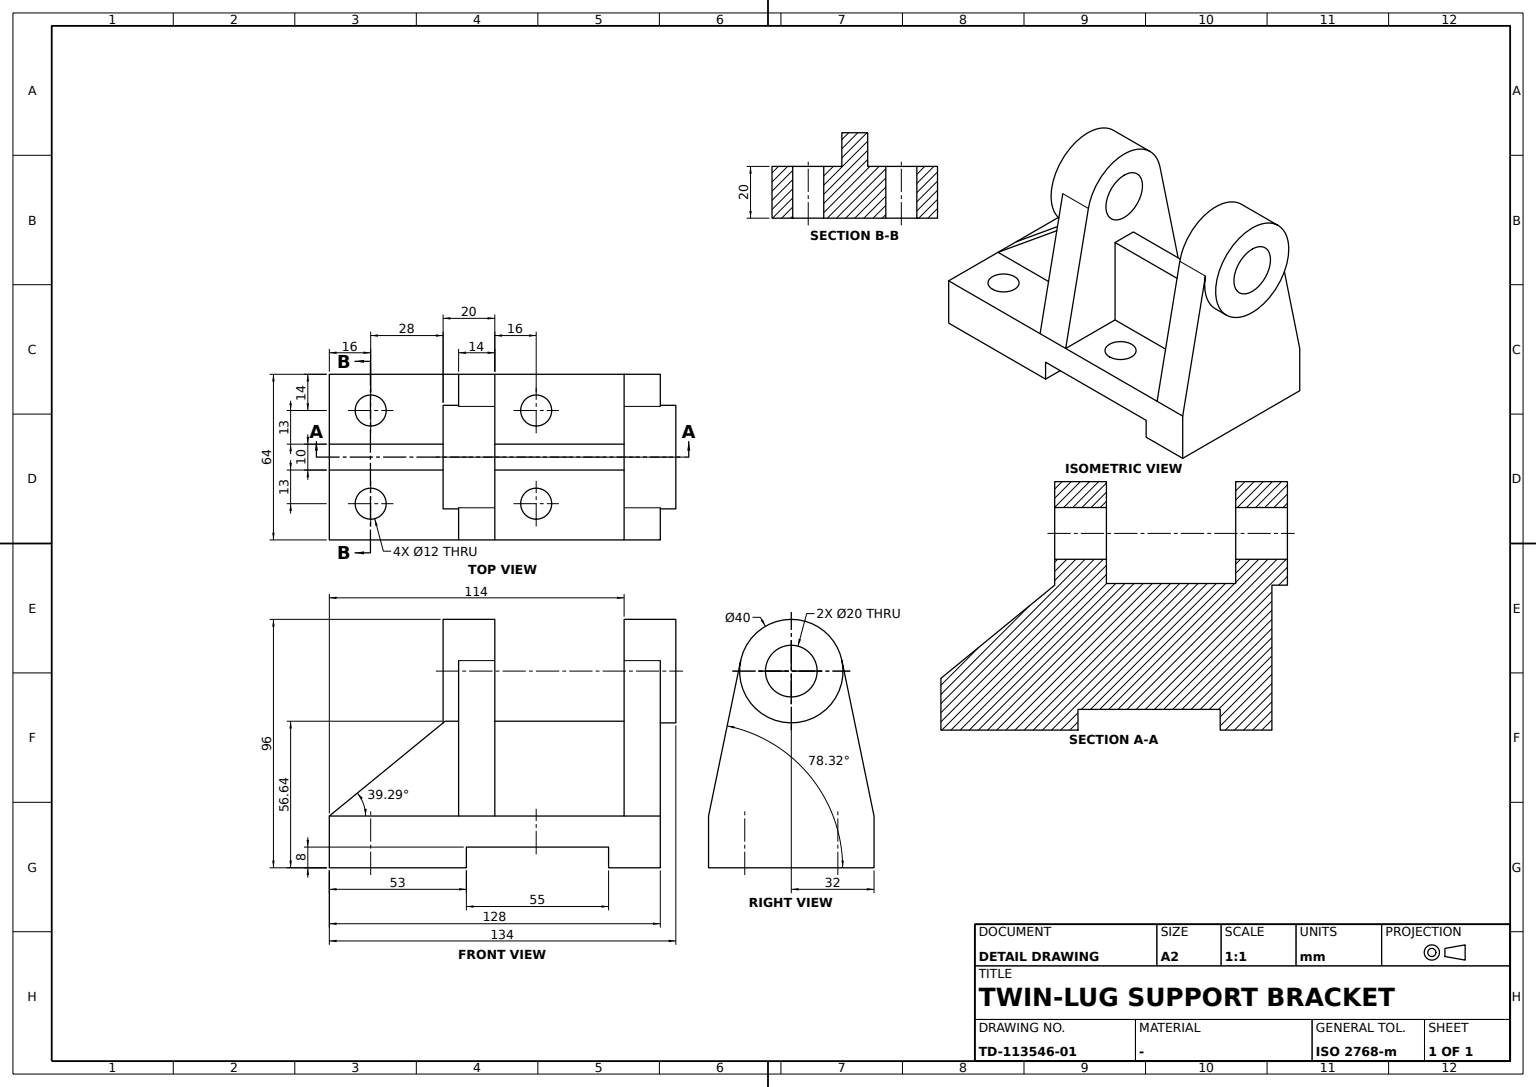
ISO-10303-21;
HEADER;
FILE_DESCRIPTION((''),'2;1');
FILE_NAME('','',(''),(''),'','','');
FILE_SCHEMA(('AUTOMOTIVE_DESIGN'));
ENDSEC;
DATA;
#1=APPLICATION_CONTEXT('');
#2=PRODUCT_CONTEXT('',#1,'mechanical');
#3=PRODUCT('','','',(#2));
#4=PRODUCT_DEFINITION_FORMATION('','',#3);
#5=PRODUCT_DEFINITION_CONTEXT('',#1,'design');
#6=PRODUCT_DEFINITION('','',#4,#5);
#7=PRODUCT_DEFINITION_SHAPE('','',#6);
#8=(LENGTH_UNIT()NAMED_UNIT(*)SI_UNIT(.MILLI.,.METRE.));
#9=(NAMED_UNIT(*)PLANE_ANGLE_UNIT()SI_UNIT($,.RADIAN.));
#10=(NAMED_UNIT(*)SI_UNIT($,.STERADIAN.)SOLID_ANGLE_UNIT());
#11=UNCERTAINTY_MEASURE_WITH_UNIT(LENGTH_MEASURE(0.005),#8,'distance_accuracy_value','');
#12=(GEOMETRIC_REPRESENTATION_CONTEXT(3)GLOBAL_UNCERTAINTY_ASSIGNED_CONTEXT((#11))GLOBAL_UNIT_ASSIGNED_CONTEXT((#8,#9,#10))REPRESENTATION_CONTEXT('',''));
#13=CARTESIAN_POINT('',(19.5858412334,50.,80.0490521334));
#14=VERTEX_POINT('',#13);
#15=CARTESIAN_POINT('',(19.5858412334,64.,80.0490521334));
#16=VERTEX_POINT('',#15);
#17=CARTESIAN_POINT('',(19.5858412334,60.,80.0490521334));
#18=DIRECTION('',(0.,1.,0.));
#19=VECTOR('',#18,1000.);
#20=LINE('',#17,#19);
#21=EDGE_CURVE('',#14,#16,#20,.T.);
#22=ORIENTED_EDGE('',*,*,#21,.T.);
#23=CARTESIAN_POINT('',(-19.5858412334,64.,80.0490521334));
#24=VERTEX_POINT('',#23);
#25=CARTESIAN_POINT('',(0.,64.,76.));
#26=DIRECTION('',(0.,0.,1.));
#27=AXIS2_PLACEMENT_3D('',#25,#18,#26);
#28=CIRCLE('',#27,20.);
#29=EDGE_CURVE('',#16,#24,#28,.T.);
#30=ORIENTED_EDGE('',*,*,#29,.T.);
#31=CARTESIAN_POINT('',(-19.5858412334,50.,80.0490521334));
#32=VERTEX_POINT('',#31);
#33=CARTESIAN_POINT('',(-19.5858412334,60.,80.0490521334));
#34=LINE('',#33,#19);
#35=EDGE_CURVE('',#32,#24,#34,.T.);
#36=ORIENTED_EDGE('',*,*,#35,.F.);
#37=CARTESIAN_POINT('',(0.,50.,76.));
#38=AXIS2_PLACEMENT_3D('',#37,#18,#26);
#39=CIRCLE('',#38,20.);
#40=EDGE_CURVE('',#32,#14,#39,.T.);
#41=ORIENTED_EDGE('',*,*,#40,.T.);
#42=EDGE_LOOP('',(#22,#30,#36,#41));
#43=FACE_BOUND('',#42,.T.);
#44=CARTESIAN_POINT('',(0.,70.,96.));
#45=VERTEX_POINT('',#44);
#46=CARTESIAN_POINT('',(0.,70.,76.));
#47=AXIS2_PLACEMENT_3D('',#46,#18,#26);
#48=CIRCLE('',#47,20.);
#49=EDGE_CURVE('',#45,#45,#48,.T.);
#50=ORIENTED_EDGE('',*,*,#49,.F.);
#51=EDGE_LOOP('',(#50));
#52=FACE_BOUND('',#51,.T.);
#53=CARTESIAN_POINT('',(0.,60.,76.));
#54=DIRECTION('',(-1.,0.,0.));
#55=AXIS2_PLACEMENT_3D('',#53,#18,#54);
#56=CYLINDRICAL_SURFACE('',#55,20.);
#57=ADVANCED_FACE('',(#43,#52),#56,.T.);
#58=CARTESIAN_POINT('',(-32.,44.,0.));
#59=VERTEX_POINT('',#58);
#60=CARTESIAN_POINT('',(32.,44.,0.));
#61=VERTEX_POINT('',#60);
#62=CARTESIAN_POINT('',(0.,44.,0.));
#63=DIRECTION('',(1.,0.,0.));
#64=VECTOR('',#63,1000.);
#65=LINE('',#62,#64);
#66=EDGE_CURVE('',#59,#61,#65,.T.);
#67=ORIENTED_EDGE('',*,*,#66,.T.);
#68=CARTESIAN_POINT('',(32.,44.,8.));
#69=VERTEX_POINT('',#68);
#70=VECTOR('',#26,1000.);
#71=LINE('',#60,#70);
#72=EDGE_CURVE('',#61,#69,#71,.T.);
#73=ORIENTED_EDGE('',*,*,#72,.T.);
#74=CARTESIAN_POINT('',(-32.,44.,8.));
#75=VERTEX_POINT('',#74);
#76=CARTESIAN_POINT('',(0.,44.,8.));
#77=LINE('',#76,#64);
#78=EDGE_CURVE('',#75,#69,#77,.T.);
#79=ORIENTED_EDGE('',*,*,#78,.F.);
#80=LINE('',#58,#70);
#81=EDGE_CURVE('',#59,#75,#80,.T.);
#82=ORIENTED_EDGE('',*,*,#81,.F.);
#83=EDGE_LOOP('',(#67,#73,#79,#82));
#84=FACE_BOUND('',#83,.T.);
#85=AXIS2_PLACEMENT_3D('',#62,#18,#26);
#86=PLANE('',#85);
#87=ADVANCED_FACE('',(#84),#86,.F.);
#88=CARTESIAN_POINT('',(-32.,-64.,20.));
#89=VERTEX_POINT('',#88);
#90=CARTESIAN_POINT('',(-32.,-64.,0.));
#91=VERTEX_POINT('',#90);
#92=DIRECTION('',(0.,0.,-1.));
#93=VECTOR('',#92,1000.);
#94=LINE('',#90,#93);
#95=EDGE_CURVE('',#89,#91,#94,.T.);
#96=ORIENTED_EDGE('',*,*,#95,.T.);
#97=CARTESIAN_POINT('',(32.,-64.,0.));
#98=VERTEX_POINT('',#97);
#99=CARTESIAN_POINT('',(0.,-64.,0.));
#100=LINE('',#99,#64);
#101=EDGE_CURVE('',#91,#98,#100,.T.);
#102=ORIENTED_EDGE('',*,*,#101,.T.);
#103=CARTESIAN_POINT('',(32.,-64.,20.));
#104=VERTEX_POINT('',#103);
#105=LINE('',#97,#93);
#106=EDGE_CURVE('',#104,#98,#105,.T.);
#107=ORIENTED_EDGE('',*,*,#106,.F.);
#108=CARTESIAN_POINT('',(5.,-64.,20.));
#109=VERTEX_POINT('',#108);
#110=CARTESIAN_POINT('',(0.,-64.,20.));
#111=LINE('',#110,#64);
#112=EDGE_CURVE('',#109,#104,#111,.T.);
#113=ORIENTED_EDGE('',*,*,#112,.F.);
#114=CARTESIAN_POINT('',(-5.,-64.,20.));
#115=VERTEX_POINT('',#114);
#116=EDGE_CURVE('',#115,#109,#111,.T.);
#117=ORIENTED_EDGE('',*,*,#116,.F.);
#118=EDGE_CURVE('',#89,#115,#111,.T.);
#119=ORIENTED_EDGE('',*,*,#118,.F.);
#120=EDGE_LOOP('',(#96,#102,#107,#113,#117,#119));
#121=FACE_BOUND('',#120,.T.);
#122=DIRECTION('',(0.,-1.,0.));
#123=AXIS2_PLACEMENT_3D('',#110,#122,#92);
#124=PLANE('',#123);
#125=ADVANCED_FACE('',(#121),#124,.T.);
#126=CARTESIAN_POINT('',(-5.,0.,20.));
#127=VERTEX_POINT('',#126);
#128=CARTESIAN_POINT('',(-32.,0.,20.));
#129=VERTEX_POINT('',#128);
#130=CARTESIAN_POINT('',(0.,0.,20.));
#131=VECTOR('',#54,1000.);
#132=LINE('',#130,#131);
#133=EDGE_CURVE('',#127,#129,#132,.T.);
#134=ORIENTED_EDGE('',*,*,#133,.F.);
#135=CARTESIAN_POINT('',(-5.,50.,20.));
#136=VERTEX_POINT('',#135);
#137=VECTOR('',#122,1000.);
#138=LINE('',#126,#137);
#139=EDGE_CURVE('',#136,#127,#138,.T.);
#140=ORIENTED_EDGE('',*,*,#139,.F.);
#141=CARTESIAN_POINT('',(-32.,50.,20.));
#142=VERTEX_POINT('',#141);
#143=CARTESIAN_POINT('',(0.,50.,20.));
#144=LINE('',#143,#131);
#145=EDGE_CURVE('',#136,#142,#144,.T.);
#146=ORIENTED_EDGE('',*,*,#145,.T.);
#147=LINE('',#128,#137);
#148=EDGE_CURVE('',#142,#129,#147,.T.);
#149=ORIENTED_EDGE('',*,*,#148,.T.);
#150=EDGE_LOOP('',(#134,#140,#146,#149));
#151=FACE_BOUND('',#150,.T.);
#152=CARTESIAN_POINT('',(-12.,16.,20.));
#153=VERTEX_POINT('',#152);
#154=CARTESIAN_POINT('',(-18.,16.,20.));
#155=AXIS2_PLACEMENT_3D('',#154,#26,#63);
#156=CIRCLE('',#155,6.);
#157=EDGE_CURVE('',#153,#153,#156,.T.);
#158=ORIENTED_EDGE('',*,*,#157,.F.);
#159=EDGE_LOOP('',(#158));
#160=FACE_BOUND('',#159,.T.);
#161=CARTESIAN_POINT('',(0.,64.,20.));
#162=AXIS2_PLACEMENT_3D('',#161,#26,#122);
#163=PLANE('',#162);
#164=ADVANCED_FACE('',(#151,#160),#163,.T.);
#165=CARTESIAN_POINT('',(-5.,-14.,56.635083269));
#166=VERTEX_POINT('',#165);
#167=CARTESIAN_POINT('',(-19.5858412334,-14.,80.0490521334));
#168=VERTEX_POINT('',#167);
#169=CARTESIAN_POINT('',(0.,-14.,76.));
#170=AXIS2_PLACEMENT_3D('',#169,#18,#26);
#171=CIRCLE('',#170,20.);
#172=EDGE_CURVE('',#166,#168,#171,.T.);
#173=ORIENTED_EDGE('',*,*,#172,.T.);
#174=CARTESIAN_POINT('',(-32.,-14.,20.));
#175=VERTEX_POINT('',#174);
#176=DIRECTION('',(-0.2024526067,0.,-0.9792920617));
#177=VECTOR('',#176,1000.);
#178=LINE('',#167,#177);
#179=EDGE_CURVE('',#168,#175,#178,.T.);
#180=ORIENTED_EDGE('',*,*,#179,.T.);
#181=CARTESIAN_POINT('',(-5.,-14.,20.));
#182=VERTEX_POINT('',#181);
#183=CARTESIAN_POINT('',(0.,-14.,20.));
#184=LINE('',#183,#131);
#185=EDGE_CURVE('',#182,#175,#184,.T.);
#186=ORIENTED_EDGE('',*,*,#185,.F.);
#187=CARTESIAN_POINT('',(-5.,-14.,0.));
#188=LINE('',#187,#93);
#189=EDGE_CURVE('',#166,#182,#188,.T.);
#190=ORIENTED_EDGE('',*,*,#189,.F.);
#191=EDGE_LOOP('',(#173,#180,#186,#190));
#192=FACE_BOUND('',#191,.T.);
#193=CARTESIAN_POINT('',(0.,-14.,0.));
#194=AXIS2_PLACEMENT_3D('',#193,#18,#54);
#195=PLANE('',#194);
#196=ADVANCED_FACE('',(#192),#195,.F.);
#197=CARTESIAN_POINT('',(-32.,-11.,0.));
#198=VERTEX_POINT('',#197);
#199=CARTESIAN_POINT('',(32.,-11.,0.));
#200=VERTEX_POINT('',#199);
#201=CARTESIAN_POINT('',(0.,-11.,0.));
#202=LINE('',#201,#64);
#203=EDGE_CURVE('',#198,#200,#202,.T.);
#204=ORIENTED_EDGE('',*,*,#203,.F.);
#205=CARTESIAN_POINT('',(-32.,-11.,8.));
#206=VERTEX_POINT('',#205);
#207=LINE('',#197,#93);
#208=EDGE_CURVE('',#206,#198,#207,.T.);
#209=ORIENTED_EDGE('',*,*,#208,.F.);
#210=CARTESIAN_POINT('',(32.,-11.,8.));
#211=VERTEX_POINT('',#210);
#212=CARTESIAN_POINT('',(0.,-11.,8.));
#213=LINE('',#212,#64);
#214=EDGE_CURVE('',#206,#211,#213,.T.);
#215=ORIENTED_EDGE('',*,*,#214,.T.);
#216=LINE('',#199,#93);
#217=EDGE_CURVE('',#211,#200,#216,.T.);
#218=ORIENTED_EDGE('',*,*,#217,.T.);
#219=EDGE_LOOP('',(#204,#209,#215,#218));
#220=FACE_BOUND('',#219,.T.);
#221=AXIS2_PLACEMENT_3D('',#212,#122,#92);
#222=PLANE('',#221);
#223=ADVANCED_FACE('',(#220),#222,.F.);
#224=CARTESIAN_POINT('',(32.,-14.,20.));
#225=VERTEX_POINT('',#224);
#226=CARTESIAN_POINT('',(32.,0.,20.));
#227=LINE('',#226,#137);
#228=EDGE_CURVE('',#225,#104,#227,.T.);
#229=ORIENTED_EDGE('',*,*,#228,.F.);
#230=CARTESIAN_POINT('',(5.,-14.,20.));
#231=VERTEX_POINT('',#230);
#232=EDGE_CURVE('',#225,#231,#184,.T.);
#233=ORIENTED_EDGE('',*,*,#232,.T.);
#234=CARTESIAN_POINT('',(5.,0.,20.));
#235=LINE('',#234,#137);
#236=EDGE_CURVE('',#231,#109,#235,.T.);
#237=ORIENTED_EDGE('',*,*,#236,.T.);
#238=ORIENTED_EDGE('',*,*,#112,.T.);
#239=EDGE_LOOP('',(#229,#233,#237,#238));
#240=FACE_BOUND('',#239,.T.);
#241=CARTESIAN_POINT('',(24.,-48.,20.));
#242=VERTEX_POINT('',#241);
#243=CARTESIAN_POINT('',(18.,-48.,20.));
#244=AXIS2_PLACEMENT_3D('',#243,#26,#63);
#245=CIRCLE('',#244,6.);
#246=EDGE_CURVE('',#242,#242,#245,.T.);
#247=ORIENTED_EDGE('',*,*,#246,.F.);
#248=EDGE_LOOP('',(#247));
#249=FACE_BOUND('',#248,.T.);
#250=ADVANCED_FACE('',(#240,#249),#163,.T.);
#251=CARTESIAN_POINT('',(32.,64.,20.));
#252=VERTEX_POINT('',#251);
#253=CARTESIAN_POINT('',(32.,50.,20.));
#254=VERTEX_POINT('',#253);
#255=LINE('',#251,#137);
#256=EDGE_CURVE('',#252,#254,#255,.T.);
#257=ORIENTED_EDGE('',*,*,#256,.F.);
#258=DIRECTION('',(0.2024526067,0.,-0.9792920617));
#259=VECTOR('',#258,1000.);
#260=LINE('',#15,#259);
#261=EDGE_CURVE('',#16,#252,#260,.T.);
#262=ORIENTED_EDGE('',*,*,#261,.F.);
#263=ORIENTED_EDGE('',*,*,#21,.F.);
#264=LINE('',#13,#259);
#265=EDGE_CURVE('',#14,#254,#264,.T.);
#266=ORIENTED_EDGE('',*,*,#265,.T.);
#267=EDGE_LOOP('',(#257,#262,#263,#266));
#268=FACE_BOUND('',#267,.T.);
#269=DIRECTION('',(-0.9792920617,0.,-0.2024526067));
#270=AXIS2_PLACEMENT_3D('',#15,#269,#258);
#271=PLANE('',#270);
#272=ADVANCED_FACE('',(#268),#271,.F.);
#273=CARTESIAN_POINT('',(-12.,16.,8.));
#274=VERTEX_POINT('',#273);
#275=CARTESIAN_POINT('',(-18.,16.,8.));
#276=AXIS2_PLACEMENT_3D('',#275,#26,#63);
#277=CIRCLE('',#276,6.);
#278=EDGE_CURVE('',#274,#274,#277,.T.);
#279=ORIENTED_EDGE('',*,*,#278,.F.);
#280=EDGE_LOOP('',(#279));
#281=FACE_BOUND('',#280,.T.);
#282=ORIENTED_EDGE('',*,*,#157,.T.);
#283=EDGE_LOOP('',(#282));
#284=FACE_BOUND('',#283,.T.);
#285=CARTESIAN_POINT('',(-18.,16.,9.));
#286=AXIS2_PLACEMENT_3D('',#285,#26,#63);
#287=CYLINDRICAL_SURFACE('',#286,6.);
#288=ADVANCED_FACE('',(#281,#284),#287,.F.);
#289=ORIENTED_EDGE('',*,*,#172,.F.);
#290=CARTESIAN_POINT('',(-5.,-19.2237871157,56.635083269));
#291=VERTEX_POINT('',#290);
#292=CARTESIAN_POINT('',(-5.,-14.0000000001,56.635083269));
#293=LINE('',#292,#19);
#294=EDGE_CURVE('',#166,#291,#293,.F.);
#295=ORIENTED_EDGE('',*,*,#294,.T.);
#296=CARTESIAN_POINT('',(0.,-20.,56.));
#297=VERTEX_POINT('',#296);
#298=CARTESIAN_POINT('',(0.,4.4444444444,76.));
#299=DIRECTION('',(0.,0.6332377903,-0.7739572992));
#300=DIRECTION('',(0.,0.7739572992,0.6332377903));
#301=AXIS2_PLACEMENT_3D('',#298,#299,#300);
#302=ELLIPSE('',#301,31.5837120079,20.);
#303=EDGE_CURVE('',#291,#297,#302,.F.);
#304=ORIENTED_EDGE('',*,*,#303,.T.);
#305=CARTESIAN_POINT('',(0.,-20.,76.));
#306=AXIS2_PLACEMENT_3D('',#305,#18,#26);
#307=CIRCLE('',#306,20.);
#308=EDGE_CURVE('',#297,#297,#307,.T.);
#309=ORIENTED_EDGE('',*,*,#308,.T.);
#310=CARTESIAN_POINT('',(5.,-19.2237871157,56.635083269));
#311=VERTEX_POINT('',#310);
#312=EDGE_CURVE('',#297,#311,#302,.F.);
#313=ORIENTED_EDGE('',*,*,#312,.T.);
#314=CARTESIAN_POINT('',(5.,-14.,56.635083269));
#315=VERTEX_POINT('',#314);
#316=CARTESIAN_POINT('',(5.,-14.0000000001,56.635083269));
#317=LINE('',#316,#19);
#318=EDGE_CURVE('',#315,#311,#317,.F.);
#319=ORIENTED_EDGE('',*,*,#318,.F.);
#320=CARTESIAN_POINT('',(19.5858412334,-14.,80.0490521334));
#321=VERTEX_POINT('',#320);
#322=EDGE_CURVE('',#321,#315,#171,.T.);
#323=ORIENTED_EDGE('',*,*,#322,.F.);
#324=CARTESIAN_POINT('',(19.5858412334,0.,80.0490521334));
#325=VERTEX_POINT('',#324);
#326=EDGE_CURVE('',#321,#325,#20,.T.);
#327=ORIENTED_EDGE('',*,*,#326,.T.);
#328=CARTESIAN_POINT('',(-19.5858412334,0.,80.0490521334));
#329=VERTEX_POINT('',#328);
#330=CARTESIAN_POINT('',(0.,0.,76.));
#331=AXIS2_PLACEMENT_3D('',#330,#18,#26);
#332=CIRCLE('',#331,20.);
#333=EDGE_CURVE('',#329,#325,#332,.T.);
#334=ORIENTED_EDGE('',*,*,#333,.F.);
#335=EDGE_CURVE('',#168,#329,#34,.T.);
#336=ORIENTED_EDGE('',*,*,#335,.F.);
#337=EDGE_LOOP('',(#289,#295,#304,#309,#313,#319,#323,#327,#334,#336));
#338=FACE_BOUND('',#337,.T.);
#339=ADVANCED_FACE('',(#338),#56,.T.);
#340=VERTEX_POINT('',#234);
#341=CARTESIAN_POINT('',(5.,0.,56.635083269));
#342=VERTEX_POINT('',#341);
#343=CARTESIAN_POINT('',(5.,0.,0.));
#344=LINE('',#343,#70);
#345=EDGE_CURVE('',#340,#342,#344,.T.);
#346=ORIENTED_EDGE('',*,*,#345,.F.);
#347=CARTESIAN_POINT('',(5.,50.,20.));
#348=VERTEX_POINT('',#347);
#349=EDGE_CURVE('',#348,#340,#235,.T.);
#350=ORIENTED_EDGE('',*,*,#349,.F.);
#351=CARTESIAN_POINT('',(5.,50.,56.635083269));
#352=VERTEX_POINT('',#351);
#353=CARTESIAN_POINT('',(5.,50.,0.));
#354=LINE('',#353,#70);
#355=EDGE_CURVE('',#348,#352,#354,.T.);
#356=ORIENTED_EDGE('',*,*,#355,.T.);
#357=LINE('',#341,#19);
#358=EDGE_CURVE('',#342,#352,#357,.T.);
#359=ORIENTED_EDGE('',*,*,#358,.F.);
#360=EDGE_LOOP('',(#346,#350,#356,#359));
#361=FACE_BOUND('',#360,.T.);
#362=AXIS2_PLACEMENT_3D('',#343,#63,#18);
#363=PLANE('',#362);
#364=ADVANCED_FACE('',(#361),#363,.T.);
#365=ORIENTED_EDGE('',*,*,#322,.T.);
#366=CARTESIAN_POINT('',(5.,-14.,0.));
#367=LINE('',#366,#93);
#368=EDGE_CURVE('',#315,#231,#367,.T.);
#369=ORIENTED_EDGE('',*,*,#368,.T.);
#370=ORIENTED_EDGE('',*,*,#232,.F.);
#371=LINE('',#320,#259);
#372=EDGE_CURVE('',#321,#225,#371,.T.);
#373=ORIENTED_EDGE('',*,*,#372,.F.);
#374=EDGE_LOOP('',(#365,#369,#370,#373));
#375=FACE_BOUND('',#374,.T.);
#376=ADVANCED_FACE('',(#375),#195,.F.);
#377=CARTESIAN_POINT('',(-12.,-48.,20.));
#378=VERTEX_POINT('',#377);
#379=CARTESIAN_POINT('',(-18.,-48.,20.));
#380=AXIS2_PLACEMENT_3D('',#379,#26,#63);
#381=CIRCLE('',#380,6.);
#382=EDGE_CURVE('',#378,#378,#381,.T.);
#383=ORIENTED_EDGE('',*,*,#382,.T.);
#384=EDGE_LOOP('',(#383));
#385=FACE_BOUND('',#384,.T.);
#386=CARTESIAN_POINT('',(-24.,-48.,0.));
#387=VERTEX_POINT('',#386);
#388=CARTESIAN_POINT('',(-18.,-48.,0.));
#389=AXIS2_PLACEMENT_3D('',#388,#92,#54);
#390=CIRCLE('',#389,6.);
#391=EDGE_CURVE('',#387,#387,#390,.T.);
#392=ORIENTED_EDGE('',*,*,#391,.T.);
#393=EDGE_LOOP('',(#392));
#394=FACE_BOUND('',#393,.T.);
#395=CARTESIAN_POINT('',(-18.,-48.,9.));
#396=AXIS2_PLACEMENT_3D('',#395,#26,#63);
#397=CYLINDRICAL_SURFACE('',#396,6.);
#398=ADVANCED_FACE('',(#385,#394),#397,.F.);
#399=CARTESIAN_POINT('',(-32.,64.,0.));
#400=VERTEX_POINT('',#399);
#401=CARTESIAN_POINT('',(-32.,0.,0.));
#402=LINE('',#401,#19);
#403=EDGE_CURVE('',#59,#400,#402,.T.);
#404=ORIENTED_EDGE('',*,*,#403,.T.);
#405=CARTESIAN_POINT('',(32.,64.,0.));
#406=VERTEX_POINT('',#405);
#407=CARTESIAN_POINT('',(0.,64.,0.));
#408=LINE('',#407,#64);
#409=EDGE_CURVE('',#400,#406,#408,.T.);
#410=ORIENTED_EDGE('',*,*,#409,.T.);
#411=CARTESIAN_POINT('',(32.,0.,0.));
#412=LINE('',#411,#19);
#413=EDGE_CURVE('',#61,#406,#412,.T.);
#414=ORIENTED_EDGE('',*,*,#413,.F.);
#415=ORIENTED_EDGE('',*,*,#66,.F.);
#416=EDGE_LOOP('',(#404,#410,#414,#415));
#417=FACE_BOUND('',#416,.T.);
#418=AXIS2_PLACEMENT_3D('',#99,#92,#18);
#419=PLANE('',#418);
#420=ADVANCED_FACE('',(#417),#419,.T.);
#421=ORIENTED_EDGE('',*,*,#49,.T.);
#422=EDGE_LOOP('',(#421));
#423=FACE_BOUND('',#422,.T.);
#424=CARTESIAN_POINT('',(0.,70.,86.));
#425=VERTEX_POINT('',#424);
#426=CIRCLE('',#47,10.);
#427=EDGE_CURVE('',#425,#425,#426,.T.);
#428=ORIENTED_EDGE('',*,*,#427,.F.);
#429=EDGE_LOOP('',(#428));
#430=FACE_BOUND('',#429,.T.);
#431=CARTESIAN_POINT('',(0.,70.,0.));
#432=AXIS2_PLACEMENT_3D('',#431,#18,#54);
#433=PLANE('',#432);
#434=ADVANCED_FACE('',(#423,#430),#433,.T.);
#435=EDGE_CURVE('',#175,#89,#147,.T.);
#436=ORIENTED_EDGE('',*,*,#435,.F.);
#437=CARTESIAN_POINT('',(-32.,64.,20.));
#438=LINE('',#437,#19);
#439=EDGE_CURVE('',#175,#129,#438,.T.);
#440=ORIENTED_EDGE('',*,*,#439,.T.);
#441=ORIENTED_EDGE('',*,*,#148,.F.);
#442=VERTEX_POINT('',#437);
#443=EDGE_CURVE('',#442,#142,#147,.T.);
#444=ORIENTED_EDGE('',*,*,#443,.F.);
#445=LINE('',#399,#70);
#446=EDGE_CURVE('',#400,#442,#445,.T.);
#447=ORIENTED_EDGE('',*,*,#446,.F.);
#448=ORIENTED_EDGE('',*,*,#403,.F.);
#449=ORIENTED_EDGE('',*,*,#81,.T.);
#450=CARTESIAN_POINT('',(-32.,0.,8.));
#451=LINE('',#450,#137);
#452=EDGE_CURVE('',#75,#206,#451,.T.);
#453=ORIENTED_EDGE('',*,*,#452,.T.);
#454=ORIENTED_EDGE('',*,*,#208,.T.);
#455=EDGE_CURVE('',#91,#198,#402,.T.);
#456=ORIENTED_EDGE('',*,*,#455,.F.);
#457=ORIENTED_EDGE('',*,*,#95,.F.);
#458=EDGE_LOOP('',(#436,#440,#441,#444,#447,#448,#449,#453,#454,#456,#457));
#459=FACE_BOUND('',#458,.T.);
#460=AXIS2_PLACEMENT_3D('',#401,#63,#18);
#461=PLANE('',#460);
#462=ADVANCED_FACE('',(#459),#461,.F.);
#463=CARTESIAN_POINT('',(5.,-20.,56.));
#464=DIRECTION('',(0.,-0.7739572992,-0.6332377903));
#465=VECTOR('',#464,1000.);
#466=LINE('',#463,#465);
#467=EDGE_CURVE('',#311,#109,#466,.T.);
#468=ORIENTED_EDGE('',*,*,#467,.F.);
#469=ORIENTED_EDGE('',*,*,#312,.F.);
#470=ORIENTED_EDGE('',*,*,#303,.F.);
#471=CARTESIAN_POINT('',(-5.,-20.,56.));
#472=LINE('',#471,#465);
#473=EDGE_CURVE('',#291,#115,#472,.T.);
#474=ORIENTED_EDGE('',*,*,#473,.T.);
#475=ORIENTED_EDGE('',*,*,#116,.T.);
#476=EDGE_LOOP('',(#468,#469,#470,#474,#475));
#477=FACE_BOUND('',#476,.T.);
#478=AXIS2_PLACEMENT_3D('',#296,#299,#300);
#479=PLANE('',#478);
#480=ADVANCED_FACE('',(#477),#479,.F.);
#481=CARTESIAN_POINT('',(12.,-48.,0.));
#482=VERTEX_POINT('',#481);
#483=CARTESIAN_POINT('',(18.,-48.,0.));
#484=AXIS2_PLACEMENT_3D('',#483,#92,#54);
#485=CIRCLE('',#484,6.);
#486=EDGE_CURVE('',#482,#482,#485,.T.);
#487=ORIENTED_EDGE('',*,*,#486,.F.);
#488=EDGE_LOOP('',(#487));
#489=FACE_BOUND('',#488,.T.);
#490=ORIENTED_EDGE('',*,*,#203,.T.);
#491=EDGE_CURVE('',#98,#200,#412,.T.);
#492=ORIENTED_EDGE('',*,*,#491,.F.);
#493=ORIENTED_EDGE('',*,*,#101,.F.);
#494=ORIENTED_EDGE('',*,*,#455,.T.);
#495=EDGE_LOOP('',(#490,#492,#493,#494));
#496=FACE_BOUND('',#495,.T.);
#497=ORIENTED_EDGE('',*,*,#391,.F.);
#498=EDGE_LOOP('',(#497));
#499=FACE_BOUND('',#498,.T.);
#500=ADVANCED_FACE('',(#489,#496,#499),#419,.T.);
#501=ORIENTED_EDGE('',*,*,#368,.F.);
#502=ORIENTED_EDGE('',*,*,#318,.T.);
#503=ORIENTED_EDGE('',*,*,#467,.T.);
#504=ORIENTED_EDGE('',*,*,#236,.F.);
#505=EDGE_LOOP('',(#501,#502,#503,#504));
#506=FACE_BOUND('',#505,.T.);
#507=ADVANCED_FACE('',(#506),#363,.T.);
#508=ORIENTED_EDGE('',*,*,#139,.T.);
#509=CARTESIAN_POINT('',(-5.,0.,56.635083269));
#510=VERTEX_POINT('',#509);
#511=CARTESIAN_POINT('',(-5.,0.,0.));
#512=LINE('',#511,#70);
#513=EDGE_CURVE('',#127,#510,#512,.T.);
#514=ORIENTED_EDGE('',*,*,#513,.T.);
#515=CARTESIAN_POINT('',(-5.,50.,56.635083269));
#516=VERTEX_POINT('',#515);
#517=LINE('',#509,#19);
#518=EDGE_CURVE('',#510,#516,#517,.T.);
#519=ORIENTED_EDGE('',*,*,#518,.T.);
#520=CARTESIAN_POINT('',(-5.,50.,0.));
#521=LINE('',#520,#70);
#522=EDGE_CURVE('',#136,#516,#521,.T.);
#523=ORIENTED_EDGE('',*,*,#522,.F.);
#524=EDGE_LOOP('',(#508,#514,#519,#523));
#525=FACE_BOUND('',#524,.T.);
#526=AXIS2_PLACEMENT_3D('',#511,#63,#18);
#527=PLANE('',#526);
#528=ADVANCED_FACE('',(#525),#527,.F.);
#529=ORIENTED_EDGE('',*,*,#427,.T.);
#530=EDGE_LOOP('',(#529));
#531=FACE_BOUND('',#530,.T.);
#532=CARTESIAN_POINT('',(0.,50.,86.));
#533=VERTEX_POINT('',#532);
#534=CIRCLE('',#38,10.);
#535=EDGE_CURVE('',#533,#533,#534,.T.);
#536=ORIENTED_EDGE('',*,*,#535,.F.);
#537=EDGE_LOOP('',(#536));
#538=FACE_BOUND('',#537,.T.);
#539=CYLINDRICAL_SURFACE('',#55,10.);
#540=ADVANCED_FACE('',(#531,#538),#539,.F.);
#541=VERTEX_POINT('',#226);
#542=LINE('',#226,#19);
#543=EDGE_CURVE('',#225,#541,#542,.T.);
#544=ORIENTED_EDGE('',*,*,#543,.T.);
#545=LINE('',#324,#259);
#546=EDGE_CURVE('',#325,#541,#545,.T.);
#547=ORIENTED_EDGE('',*,*,#546,.F.);
#548=ORIENTED_EDGE('',*,*,#326,.F.);
#549=ORIENTED_EDGE('',*,*,#372,.T.);
#550=EDGE_LOOP('',(#544,#547,#548,#549));
#551=FACE_BOUND('',#550,.T.);
#552=ADVANCED_FACE('',(#551),#271,.F.);
#553=ORIENTED_EDGE('',*,*,#246,.T.);
#554=EDGE_LOOP('',(#553));
#555=FACE_BOUND('',#554,.T.);
#556=ORIENTED_EDGE('',*,*,#486,.T.);
#557=EDGE_LOOP('',(#556));
#558=FACE_BOUND('',#557,.T.);
#559=CARTESIAN_POINT('',(18.,-48.,9.));
#560=AXIS2_PLACEMENT_3D('',#559,#26,#63);
#561=CYLINDRICAL_SURFACE('',#560,6.);
#562=ADVANCED_FACE('',(#555,#558),#561,.F.);
#563=ORIENTED_EDGE('',*,*,#185,.T.);
#564=ORIENTED_EDGE('',*,*,#435,.T.);
#565=ORIENTED_EDGE('',*,*,#118,.T.);
#566=EDGE_CURVE('',#182,#115,#138,.T.);
#567=ORIENTED_EDGE('',*,*,#566,.F.);
#568=EDGE_LOOP('',(#563,#564,#565,#567));
#569=FACE_BOUND('',#568,.T.);
#570=ORIENTED_EDGE('',*,*,#382,.F.);
#571=EDGE_LOOP('',(#570));
#572=FACE_BOUND('',#571,.T.);
#573=ADVANCED_FACE('',(#569,#572),#163,.T.);
#574=LINE('',#328,#177);
#575=EDGE_CURVE('',#329,#129,#574,.T.);
#576=ORIENTED_EDGE('',*,*,#575,.T.);
#577=ORIENTED_EDGE('',*,*,#439,.F.);
#578=ORIENTED_EDGE('',*,*,#179,.F.);
#579=ORIENTED_EDGE('',*,*,#335,.T.);
#580=EDGE_LOOP('',(#576,#577,#578,#579));
#581=FACE_BOUND('',#580,.T.);
#582=DIRECTION('',(-0.9792920617,0.,0.2024526067));
#583=AXIS2_PLACEMENT_3D('',#23,#582,#176);
#584=PLANE('',#583);
#585=ADVANCED_FACE('',(#581),#584,.T.);
#586=EDGE_CURVE('',#254,#541,#227,.T.);
#587=ORIENTED_EDGE('',*,*,#586,.T.);
#588=ORIENTED_EDGE('',*,*,#543,.F.);
#589=ORIENTED_EDGE('',*,*,#228,.T.);
#590=ORIENTED_EDGE('',*,*,#106,.T.);
#591=ORIENTED_EDGE('',*,*,#491,.T.);
#592=ORIENTED_EDGE('',*,*,#217,.F.);
#593=CARTESIAN_POINT('',(32.,0.,8.));
#594=LINE('',#593,#137);
#595=EDGE_CURVE('',#69,#211,#594,.T.);
#596=ORIENTED_EDGE('',*,*,#595,.F.);
#597=ORIENTED_EDGE('',*,*,#72,.F.);
#598=ORIENTED_EDGE('',*,*,#413,.T.);
#599=LINE('',#405,#70);
#600=EDGE_CURVE('',#406,#252,#599,.T.);
#601=ORIENTED_EDGE('',*,*,#600,.T.);
#602=ORIENTED_EDGE('',*,*,#256,.T.);
#603=EDGE_LOOP('',(#587,#588,#589,#590,#591,#592,#596,#597,#598,#601,#602));
#604=FACE_BOUND('',#603,.T.);
#605=AXIS2_PLACEMENT_3D('',#411,#63,#18);
#606=PLANE('',#605);
#607=ADVANCED_FACE('',(#604),#606,.T.);
#608=ORIENTED_EDGE('',*,*,#473,.F.);
#609=ORIENTED_EDGE('',*,*,#294,.F.);
#610=ORIENTED_EDGE('',*,*,#189,.T.);
#611=ORIENTED_EDGE('',*,*,#566,.T.);
#612=EDGE_LOOP('',(#608,#609,#610,#611));
#613=FACE_BOUND('',#612,.T.);
#614=ADVANCED_FACE('',(#613),#527,.F.);
#615=CARTESIAN_POINT('',(0.,-20.,86.));
#616=VERTEX_POINT('',#615);
#617=CIRCLE('',#306,10.);
#618=EDGE_CURVE('',#616,#616,#617,.T.);
#619=ORIENTED_EDGE('',*,*,#618,.F.);
#620=EDGE_LOOP('',(#619));
#621=FACE_BOUND('',#620,.T.);
#622=CARTESIAN_POINT('',(0.,0.,86.));
#623=VERTEX_POINT('',#622);
#624=CIRCLE('',#331,10.);
#625=EDGE_CURVE('',#623,#623,#624,.T.);
#626=ORIENTED_EDGE('',*,*,#625,.T.);
#627=EDGE_LOOP('',(#626));
#628=FACE_BOUND('',#627,.T.);
#629=ADVANCED_FACE('',(#621,#628),#539,.F.);
#630=ORIENTED_EDGE('',*,*,#333,.T.);
#631=ORIENTED_EDGE('',*,*,#546,.T.);
#632=EDGE_CURVE('',#541,#340,#132,.T.);
#633=ORIENTED_EDGE('',*,*,#632,.T.);
#634=ORIENTED_EDGE('',*,*,#345,.T.);
#635=CARTESIAN_POINT('',(0.,0.,56.635083269));
#636=LINE('',#635,#131);
#637=EDGE_CURVE('',#342,#510,#636,.T.);
#638=ORIENTED_EDGE('',*,*,#637,.T.);
#639=ORIENTED_EDGE('',*,*,#513,.F.);
#640=ORIENTED_EDGE('',*,*,#133,.T.);
#641=ORIENTED_EDGE('',*,*,#575,.F.);
#642=EDGE_LOOP('',(#630,#631,#633,#634,#638,#639,#640,#641));
#643=FACE_BOUND('',#642,.T.);
#644=ORIENTED_EDGE('',*,*,#625,.F.);
#645=EDGE_LOOP('',(#644));
#646=FACE_BOUND('',#645,.T.);
#647=CARTESIAN_POINT('',(0.,0.,0.));
#648=AXIS2_PLACEMENT_3D('',#647,#18,#54);
#649=PLANE('',#648);
#650=ADVANCED_FACE('',(#643,#646),#649,.T.);
#651=LINE('',#23,#177);
#652=EDGE_CURVE('',#24,#442,#651,.T.);
#653=ORIENTED_EDGE('',*,*,#652,.T.);
#654=ORIENTED_EDGE('',*,*,#443,.T.);
#655=LINE('',#31,#177);
#656=EDGE_CURVE('',#32,#142,#655,.T.);
#657=ORIENTED_EDGE('',*,*,#656,.F.);
#658=ORIENTED_EDGE('',*,*,#35,.T.);
#659=EDGE_LOOP('',(#653,#654,#657,#658));
#660=FACE_BOUND('',#659,.T.);
#661=ADVANCED_FACE('',(#660),#584,.T.);
#662=ORIENTED_EDGE('',*,*,#446,.T.);
#663=ORIENTED_EDGE('',*,*,#652,.F.);
#664=ORIENTED_EDGE('',*,*,#29,.F.);
#665=ORIENTED_EDGE('',*,*,#261,.T.);
#666=ORIENTED_EDGE('',*,*,#600,.F.);
#667=ORIENTED_EDGE('',*,*,#409,.F.);
#668=EDGE_LOOP('',(#662,#663,#664,#665,#666,#667));
#669=FACE_BOUND('',#668,.T.);
#670=AXIS2_PLACEMENT_3D('',#407,#18,#26);
#671=PLANE('',#670);
#672=ADVANCED_FACE('',(#669),#671,.T.);
#673=ORIENTED_EDGE('',*,*,#308,.F.);
#674=EDGE_LOOP('',(#673));
#675=FACE_BOUND('',#674,.T.);
#676=ORIENTED_EDGE('',*,*,#618,.T.);
#677=EDGE_LOOP('',(#676));
#678=FACE_BOUND('',#677,.T.);
#679=CARTESIAN_POINT('',(0.,-20.,0.));
#680=AXIS2_PLACEMENT_3D('',#679,#18,#54);
#681=PLANE('',#680);
#682=ADVANCED_FACE('',(#675,#678),#681,.F.);
#683=ORIENTED_EDGE('',*,*,#535,.T.);
#684=EDGE_LOOP('',(#683));
#685=FACE_BOUND('',#684,.T.);
#686=ORIENTED_EDGE('',*,*,#656,.T.);
#687=ORIENTED_EDGE('',*,*,#145,.F.);
#688=ORIENTED_EDGE('',*,*,#522,.T.);
#689=CARTESIAN_POINT('',(0.,50.,56.635083269));
#690=LINE('',#689,#131);
#691=EDGE_CURVE('',#352,#516,#690,.T.);
#692=ORIENTED_EDGE('',*,*,#691,.F.);
#693=ORIENTED_EDGE('',*,*,#355,.F.);
#694=EDGE_CURVE('',#254,#348,#144,.T.);
#695=ORIENTED_EDGE('',*,*,#694,.F.);
#696=ORIENTED_EDGE('',*,*,#265,.F.);
#697=ORIENTED_EDGE('',*,*,#40,.F.);
#698=EDGE_LOOP('',(#686,#687,#688,#692,#693,#695,#696,#697));
#699=FACE_BOUND('',#698,.T.);
#700=CARTESIAN_POINT('',(0.,50.,0.));
#701=AXIS2_PLACEMENT_3D('',#700,#18,#54);
#702=PLANE('',#701);
#703=ADVANCED_FACE('',(#685,#699),#702,.F.);
#704=ORIENTED_EDGE('',*,*,#518,.F.);
#705=ORIENTED_EDGE('',*,*,#637,.F.);
#706=ORIENTED_EDGE('',*,*,#358,.T.);
#707=ORIENTED_EDGE('',*,*,#691,.T.);
#708=EDGE_LOOP('',(#704,#705,#706,#707));
#709=FACE_BOUND('',#708,.T.);
#710=AXIS2_PLACEMENT_3D('',#635,#26,#122);
#711=PLANE('',#710);
#712=ADVANCED_FACE('',(#709),#711,.T.);
#713=CARTESIAN_POINT('',(24.,16.,20.));
#714=VERTEX_POINT('',#713);
#715=CARTESIAN_POINT('',(18.,16.,20.));
#716=AXIS2_PLACEMENT_3D('',#715,#26,#63);
#717=CIRCLE('',#716,6.);
#718=EDGE_CURVE('',#714,#714,#717,.T.);
#719=ORIENTED_EDGE('',*,*,#718,.T.);
#720=EDGE_LOOP('',(#719));
#721=FACE_BOUND('',#720,.T.);
#722=CARTESIAN_POINT('',(24.,16.,8.));
#723=VERTEX_POINT('',#722);
#724=CARTESIAN_POINT('',(18.,16.,8.));
#725=AXIS2_PLACEMENT_3D('',#724,#26,#63);
#726=CIRCLE('',#725,6.);
#727=EDGE_CURVE('',#723,#723,#726,.T.);
#728=ORIENTED_EDGE('',*,*,#727,.F.);
#729=EDGE_LOOP('',(#728));
#730=FACE_BOUND('',#729,.T.);
#731=CARTESIAN_POINT('',(18.,16.,9.));
#732=AXIS2_PLACEMENT_3D('',#731,#26,#63);
#733=CYLINDRICAL_SURFACE('',#732,6.);
#734=ADVANCED_FACE('',(#721,#730),#733,.F.);
#735=ORIENTED_EDGE('',*,*,#278,.T.);
#736=EDGE_LOOP('',(#735));
#737=FACE_BOUND('',#736,.T.);
#738=ORIENTED_EDGE('',*,*,#727,.T.);
#739=EDGE_LOOP('',(#738));
#740=FACE_BOUND('',#739,.T.);
#741=ORIENTED_EDGE('',*,*,#214,.F.);
#742=ORIENTED_EDGE('',*,*,#452,.F.);
#743=ORIENTED_EDGE('',*,*,#78,.T.);
#744=ORIENTED_EDGE('',*,*,#595,.T.);
#745=EDGE_LOOP('',(#741,#742,#743,#744));
#746=FACE_BOUND('',#745,.T.);
#747=AXIS2_PLACEMENT_3D('',#76,#26,#122);
#748=PLANE('',#747);
#749=ADVANCED_FACE('',(#737,#740,#746),#748,.F.);
#750=ORIENTED_EDGE('',*,*,#718,.F.);
#751=EDGE_LOOP('',(#750));
#752=FACE_BOUND('',#751,.T.);
#753=ORIENTED_EDGE('',*,*,#694,.T.);
#754=ORIENTED_EDGE('',*,*,#349,.T.);
#755=ORIENTED_EDGE('',*,*,#632,.F.);
#756=ORIENTED_EDGE('',*,*,#586,.F.);
#757=EDGE_LOOP('',(#753,#754,#755,#756));
#758=FACE_BOUND('',#757,.T.);
#759=ADVANCED_FACE('',(#752,#758),#163,.T.);
#760=CLOSED_SHELL('',(#57,#87,#125,#164,#196,#223,#250,#272,#288,#339,#364,#376,#398,#420,#434,#462,#480,#500,#507,#528,#540,#552,#562,#573,#585,#607,#614,#629,#650,#661,#672,#682,#703,#712,#734,#749,#759));
#761=MANIFOLD_SOLID_BREP('',#760);
#762=ADVANCED_BREP_SHAPE_REPRESENTATION('',(#761),#12);
#763=SHAPE_DEFINITION_REPRESENTATION(#7,#762);
ENDSEC;
END-ISO-10303-21;
